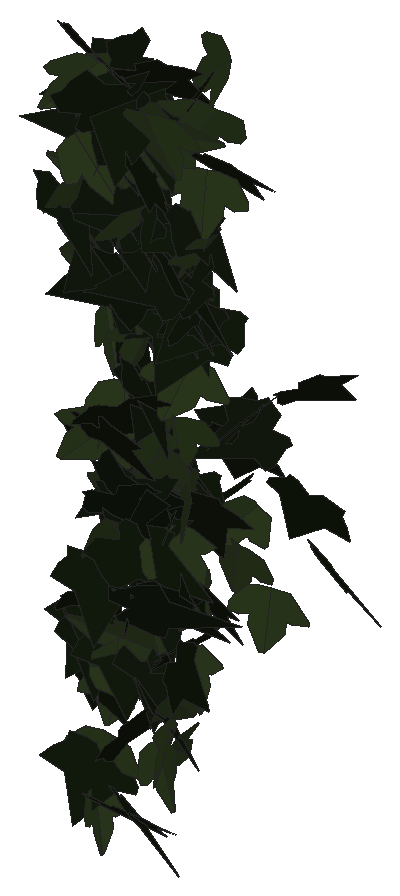
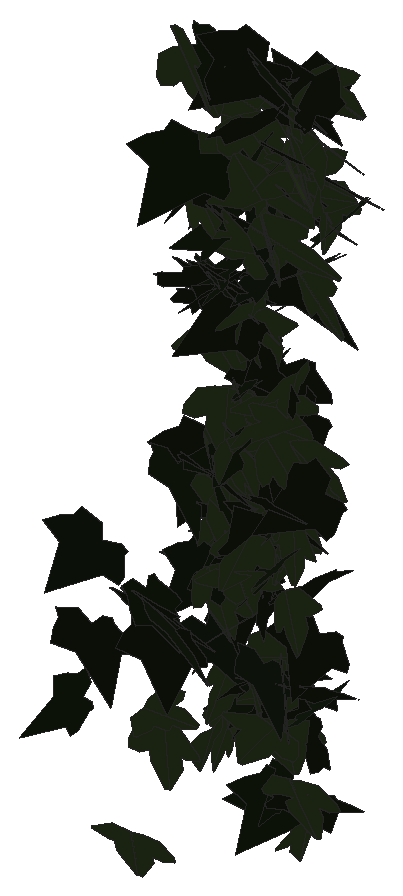
# SketchUp Ruby script. Lengths in inches.
U = 1.inch
M = Sketchup.active_model
def pt(a) = Geom::Point3d.new(a.map { |v| v * U })
def face(e, loops, mat)
  f = e.add_face(loops[0].map { |a| pt(a) })
  loops[1..].each { |l| e.add_face(l.map { |a| pt(a) }).erase! }
  f.material = f.back_material = mat if mat
  f
end
# faces: each face lists its corners as indices into pts; further lists are holes
def faces(e, pts, list, mat = nil) = list.each { |f| face(e, (f[0].is_a?(Array) ? f : [f]).map { |l| l.map { |i| pts[i] } }, mat) }
# xy, xz, yz: faces in a plane at the given z, y or x. An outline is a flat list of corners, or four numbers for a rectangle; further outlines are holes
def ring(l) = l.size == 4 ? [[l[0], l[1]], [l[2], l[1]], [l[2], l[3]], [l[0], l[3]]] : l.each_slice(2).to_a
def flat(e, list, mat, &to3) = list.each { |f| face(e, (f[0].is_a?(Array) ? f : [f]).map { |l| ring(l).map { |u, v| to3.(u, v) } }, mat) }
def xy(e, z, list, mat = nil) = flat(e, list, mat) { |x, y| [x, y, z] }
def xz(e, y, list, mat = nil) = flat(e, list, mat) { |x, z| [x, y, z] }
def yz(e, x, list, mat = nil) = flat(e, list, mat) { |y, z| [x, y, z] }
def lines(e, pts, list) = list.each { |a, b| e.add_line(pt(pts[a]), pt(pts[b])) }
# prism: a flat outline (further loops are holes) pulled along v
def prism(e, loops, v, mat = nil)
  f = face(e, loops, mat); d = Geom::Vector3d.new(v.map { |x| x * U })
  f.pushpull(f.normal.samedirection?(d) ? d.length : -d.length)
end
def box(e, o, s, mat = nil) = prism(e, [[o, [o[0] + s[0], o[1], o[2]], [o[0] + s[0], o[1] + s[1], o[2]], [o[0], o[1] + s[1], o[2]]]], [0, 0, s[2]], mat)
def at(x, y, z, deg = 0) = Geom::Transformation.translation(pt([x, y, z])) * Geom::Transformation.rotation(ORIGIN, Z_AXIS, deg.degrees)
def axes(o, x, y, z) = Geom::Transformation.new([*x, 0, *y, 0, *z, 0, *pt(o).to_a, 1])
def part(name) = M.definitions.add(name)
# library, detail: a bought-in or finely detailed component or shape, given as its bounding box
def library(name, o, s) = part(name).tap { |d| box(d.entities, o, s) }
def detail(e, o, s) = box(e.add_group.entities, o, s)
def put(e, d, t, mat = nil) = e.add_instance(d, t).tap { |i| i.material = mat if mat }
def group(e, t, mat = nil) = e.add_group.tap { |g| g.transformation = t; g.material = mat if mat }.entities
root = M.entities
M.materials.add("1026 AP 7946 SUNNY SIDE UP").color = [254, 231, 186]
M.materials.add("efeu1").color = [18, 25, 13]
M.materials.add("efeu2").color = [43, 57, 29]
c1 = part("ivyleaf_10")
p = [[0,0.5,-0.03],[-0.0625,2.02,-0.43],[-0.19,2.01,-0.46],[-0.54,1.05,-0.29],[-0.52,0.625,-0.18],[-0.83,0.76,-0.28],
  [-1.16,0.64,-0.33],[-1.15,0.33,-0.24],[-0.77,-0.39,0.02],[-0.3,-0.51,0.16],[0.04,-0.48,0.23],[-0.02,2.01,-0.4375],
  [-0.06,2.01,-0.43],[0.04,-0.49,0.23],[0.67,-0.49,0.14],[1.38,0.36,-0.2],[1.375,0.51,-0.24],[0.81,0.65,-0.19],
  [0.62,0.59,-0.15],[0.6,1.09,-0.28],[0.5,1.23,-0.31]]
faces(c1.entities,p,[[0,1,2,3,4,5,6,7,8,9,10],[11,12,0,13,14,15,16,17,18,19,20]],"efeu2")
c2 = part("ivyleaf_9")
p = [[1.54,2.16,1.25],[1.36,2.04,1.19],[-0.21,0.99,0.68],[-0.71,1.11,0.82],[-0.85,0.86,0.67],[-0.8,0.17,0.21],
  [-0.9,-0.01,0.1],[-0.67,-0.16,-0.02],[-0.08,-0.08,-0.05],[-0.03,-0.6,-0.4],[0.65,-0.88,-0.66],[0.83,-0.6,-0.49],
  [1.29,-0.42,-0.43],[1.8125,-0.07,-0.26],[1.21,0.44,0.15]]
faces(c2.entities,p,[[0,1,2,3,4,5,6,7,8,9,10,11,12,13,14]],"efeu1")
put(root,c1,axes([136.3125,212.4,287.8],[0.22711,-0.11423,-0.31893],[-0.31523,0.23716,-0.18551],[0.41092,0.24506,0.03395]),"1026 AP 7946 SUNNY SIDE UP")
put(root,c2,axes([136.11,212.92,282.05],[-0.39568,-0.19677,-0.00291],[0.06839,-0.05292,-0.32174],[0.30176,-0.24602,0.0691]),"1026 AP 7946 SUNNY SIDE UP")
put(root,c2,axes([135.93,212.8,281.74],[-0.01762,-0.28672,0.14922],[0.03799,-0.1469,-0.29519],[0.50484,0.00105,0.02742]),"1026 AP 7946 SUNNY SIDE UP")
put(root,c2,axes([136.11,212.5,282.66],[0.19885,0.2925,0.05494],[0.06419,0.03851,-0.32729],[-0.46262,0.13107,-0.0218]),"1026 AP 7946 SUNNY SIDE UP")
put(root,c2,axes([136.56,212.64,289.74],[-0.41749,0.17956,0.16578],[-0.29275,-0.0028,-0.31525],[-0.23923,-0.30993,0.09647]),"1026 AP 7946 SUNNY SIDE UP")
put(root,c2,axes([136.4375,215.3,284.04],[-0.17558,0.27212,0.14792],[-0.13121,0.11854,-0.30085],[-0.46449,-0.13635,0.02907]),"1026 AP 7946 SUNNY SIDE UP")
put(root,c1,axes([136.02,212.76,290.125],[-0.38951,0.18272,-0.18147],[0.16298,-0.1534,-0.31315],[-0.36553,-0.26311,0.05375]),"1026 AP 7946 SUNNY SIDE UP")
put(root,c2,axes([136.35,212.9375,282.23],[0.0418,-0.02393,-0.32843],[-0.44677,0.14457,-0.03476],[0.22996,0.28523,-0.00783]),"1026 AP 7946 SUNNY SIDE UP")
put(root,c2,axes([135.87,212.71,284.94],[0.55171,-0.05991,0.00291],[-0.0043,-0.03472,-0.36515],[0.09424,0.34916,-0.03369]),"1026 AP 7946 SUNNY SIDE UP")
put(root,c2,axes([135.95,212.21,288.77],[0.13325,-0.34559,0.0192],[-0.00393,-0.02182,-0.36662],[0.54436,0.08444,-0.00734]),"1026 AP 7946 SUNNY SIDE UP")
put(root,c1,axes([136.2,212.11,289.04],[-0.0567,-0.33283,-0.13417],[0.05703,0.12491,-0.34347],[0.558,-0.04658,0.02147]),"1026 AP 7946 SUNNY SIDE UP")
put(root,c2,axes([136.57,212.78,290.51],[-0.50445,0.15238,0.04087],[-0.09305,-0.0353,-0.36136],[-0.22907,-0.32122,0.05677]),"1026 AP 7946 SUNNY SIDE UP")
put(root,c1,axes([136.38,212.21,290.72],[0.30855,0.18135,-0.23522],[-0.30332,-0.12727,-0.27444],[-0.3455,0.27369,0.03088]),"1026 AP 7946 SUNNY SIDE UP")
put(root,c1,axes([136.21,212.88,286.625],[0.04732,0.33528,-0.05256],[-0.00894,-0.05263,-0.3471],[-0.53365,0.03061,0.00116]),"1026 AP 7946 SUNNY SIDE UP")
put(root,c2,axes([135.9375,212.75,281.33],[0.06984,-0.05533,-0.32343],[0.49967,-0.01336,0.04871],[-0.0333,-0.31648,0.05258]),"1026 AP 7946 SUNNY SIDE UP")
put(root,c2,axes([136.31,212.5625,280.15],[-0.35995,-0.22147,-0.03792],[0.05886,0.01237,-0.32759],[0.34775,-0.23133,0.01619]),"1026 AP 7946 SUNNY SIDE UP")
put(root,c1,axes([136.45,212.43,285.25],[0.45702,0.00054,-0.18527],[-0.28272,0.0078,-0.2993],[0.00573,0.3417,0.00912]),"1026 AP 7946 SUNNY SIDE UP")
put(root,c2,axes([136.38,215.33,283.78],[0.36414,0.10931,-0.20524],[-0.29646,-0.06793,-0.26376],[-0.20098,0.29825,0.01721]),"1026 AP 7946 SUNNY SIDE UP")
put(root,c1,axes([136.43,212.68,284.16],[-0.45237,0.14785,0.07414],[-0.13808,-0.01749,-0.32859],[-0.21792,-0.29584,0.05431]),"1026 AP 7946 SUNNY SIDE UP")
put(root,c1,axes([136.36,212.77,283.15],[-0.05788,-0.32062,-0.01386],[0.01286,0.01077,-0.33233],[0.5043,-0.03707,0.00688]),"1026 AP 7946 SUNNY SIDE UP")
put(root,c1,axes([136.34,212.64,280.33],[0.48967,-0.00134,-0.07543],[-0.11421,0.0349,-0.31874],[0.0146,0.318,0.03655]),"1026 AP 7946 SUNNY SIDE UP")
put(root,c2,axes([136,212.71,290.64],[0.02921,-0.17516,0.31941],[0.26543,-0.27013,-0.16868],[0.49458,0.15532,0.07166]),"1026 AP 7946 SUNNY SIDE UP")
put(root,c2,axes([136.53,213.08,282.3],[-0.0458,0.31236,0.06995],[-0.01903,0.06527,-0.32275],[-0.50169,-0.03099,0.00586]),"1026 AP 7946 SUNNY SIDE UP")
put(root,c1,axes([136.37,212.65,289.99],[0.29784,-0.30633,-0.0179],[0.01599,0.02464,-0.37023],[0.48204,0.18846,0.02334]),"1026 AP 7946 SUNNY SIDE UP")
put(root,c1,axes([136.82,212.36,289.03],[-0.10399,-0.03302,-0.37806],[-0.57717,0.03614,0.06504],[0.04697,0.37095,-0.03778]),"1026 AP 7946 SUNNY SIDE UP")
put(root,c1,axes([136.3125,212.61,290.47],[0.00072,-0.11466,0.35277],[0.1722,-0.32694,-0.11462],[0.5421,0.10401,0.03594]),"1026 AP 7946 SUNNY SIDE UP")
put(root,c1,axes([136.78,212.65,288.48],[0.20804,-0.05926,-0.35938],[-0.53558,0.07823,-0.14646],[0.14878,0.36448,-0.0247]),"1026 AP 7946 SUNNY SIDE UP")
put(root,c1,axes([136.55,215.2,282.19],[-0.4989,0.05063,0.08616],[-0.13581,-0.01421,-0.32994],[-0.07119,-0.32774,0.02565]),"1026 AP 7946 SUNNY SIDE UP")
put(root,c1,axes([136.4,212.8,281.29],[0.39938,0.19612,-0.03382],[-0.08539,0.01534,-0.32721],[-0.30108,0.25579,0.04794]),"1026 AP 7946 SUNNY SIDE UP")
put(root,c1,axes([136.54,215.4,282.68],[0.18051,0.15225,-0.26543],[-0.24645,-0.20559,-0.19764],[-0.40226,0.19428,0.00198]),"1026 AP 7946 SUNNY SIDE UP")
put(root,c1,axes([136.2,213.4,281.5625],[0.41864,0.08276,0.15999],[0.2167,0.07574,-0.28538],[-0.17103,0.29853,0.03004]),"1026 AP 7946 SUNNY SIDE UP")
put(root,c1,axes([136.47,212.58,289.62],[0.23919,-0.31924,0.07365],[0.02174,-0.07449,-0.36421],[0.51458,0.15154,-0.01885]),"1026 AP 7946 SUNNY SIDE UP")
put(root,c1,axes([136.375,216,281.06],[0.50983,0.03135,0.03273],[0.0544,-0.03145,-0.33388],[-0.04402,0.32425,-0.03362]),"1026 AP 7946 SUNNY SIDE UP")
put(root,c1,axes([136.4375,212.36,279.63],[0.04171,0.31122,-0.0649],[-0.0065,-0.06465,-0.32215],[-0.4998,0.02681,-0.00123]),"1026 AP 7946 SUNNY SIDE UP")
put(root,c2,axes([136.53,212.49,287.9],[-0.28062,-0.21055,0.21638],[-0.05922,-0.22828,-0.26853],[0.46521,-0.15606,0.09634]),"1026 AP 7946 SUNNY SIDE UP")
put(root,c1,axes([136.89,212.55,282.11],[-0.15009,0.0224,-0.32404],[-0.49191,-0.04909,0.09387],[-0.06393,0.32515,0.03845]),"1026 AP 7946 SUNNY SIDE UP")
put(root,c2,axes([136.72,215.27,284.32],[-0.1906,0.28286,-0.11514],[0.04144,-0.11182,-0.3171],[-0.47737,-0.12265,0.01844]),"1026 AP 7946 SUNNY SIDE UP")
put(root,c2,axes([136.89,212.25,287.76],[0.08438,-0.00333,-0.37536],[-0.51526,-0.16145,-0.04914],[-0.25048,0.331,-0.02535]),"1026 AP 7946 SUNNY SIDE UP")
put(root,c1,axes([136.38,212.15,289.58],[0.23375,0.32418,0.14353],[0.11799,0.11664,-0.36624],[-0.54097,0.16552,-0.01786]),"1026 AP 7946 SUNNY SIDE UP")
put(root,c1,axes([136.66,212.6875,285.29],[-0.14496,-0.30093,0.13342],[-0.02274,-0.13244,-0.32414],[0.5157,-0.09043,0.02321]),"1026 AP 7946 SUNNY SIDE UP")
put(root,c2,axes([136.51,212.27,283.17],[-0.11539,-0.32614,0.0352],[-0.00514,-0.03618,-0.34457],[0.51592,-0.07331,0.00444]),"1026 AP 7946 SUNNY SIDE UP")
put(root,c2,axes([136.4,212.85,283.83],[0.17585,-0.31037,0.00954],[0.00809,-0.00986,-0.33992],[0.48827,0.11194,0.0022]),"1026 AP 7946 SUNNY SIDE UP")
put(root,c2,axes([136.88,212.81,284.51],[-0.51971,-0.00684,0.00555],[-0.00759,-0.02808,-0.33952],[0.01144,-0.32937,0.02689]),"1026 AP 7946 SUNNY SIDE UP")
put(root,c2,axes([136.96,215.29,284.15],[-0.51099,0.04314,0.051],[-0.08307,-0.02544,-0.33628],[-0.06082,-0.3277,0.03086]),"1026 AP 7946 SUNNY SIDE UP")
put(root,c2,axes([136.88,212.65,290.91],[-0.49048,0.15024,-0.11639],[0.12366,-0.09628,-0.35351],[-0.26936,-0.31778,0.04964]),"1026 AP 7946 SUNNY SIDE UP")
put(root,c1,axes([136.69,212.27,284.03],[-0.07167,-0.3198,-0.2423],[0.08889,0.22726,-0.33086],[0.61614,-0.06999,0.01955]),"1026 AP 7946 SUNNY SIDE UP")
put(root,c2,axes([136.51,212.46,290.5],[-0.31983,-0.12909,-0.27626],[0.43459,0.03623,-0.23437],[0.17075,-0.33403,0.07907]),"1026 AP 7946 SUNNY SIDE UP")
put(root,c1,axes([136.54,212.41,281.68],[-0.00004,0.04067,0.34352],[0.1383,0.32158,-0.03854],[-0.5094,0.0873,-0.01049]),"1026 AP 7946 SUNNY SIDE UP")
put(root,c1,axes([136.77,212.73,288.61],[0.20674,-0.32517,-0.03944],[0.00088,0.0395,-0.36076],[0.5145,0.13059,0.01646]),"1026 AP 7946 SUNNY SIDE UP")
put(root,c2,axes([136.64,212.64,281.97],[-0.20693,-0.28592,-0.07174],[0.106,0.04317,-0.32108],[0.44981,-0.14171,0.04266]),"1026 AP 7946 SUNNY SIDE UP")
put(root,c2,axes([136.51,212.59,289.77],[0.25727,-0.37368,-0.10031],[-0.08449,0.08037,-0.41943],[0.60045,0.17141,-0.01604]),"1026 AP 7946 SUNNY SIDE UP")
put(root,c2,axes([136.53,212.83,286.61],[-0.13587,-0.03758,-0.33807],[0.51895,-0.00347,-0.08919],[0.00975,-0.33912,0.03637]),"1026 AP 7946 SUNNY SIDE UP")
put(root,c2,axes([136.53,211.95,290.28],[0.03045,0.02938,0.3747],[0.54116,0.11908,-0.0281],[-0.18991,0.34404,-0.02]),"1026 AP 7946 SUNNY SIDE UP")
put(root,c2,axes([136.63,212.52,284.25],[0.21093,-0.30298,0.00086],[-0.01608,-0.00732,-0.34116],[0.47614,0.13397,-0.0119]),"1026 AP 7946 SUNNY SIDE UP")
put(root,c1,axes([136.79,212.46,285.87],[0.39465,0.22971,-0.04215],[-0.02282,-0.04651,-0.34988],[-0.36653,0.25023,-0.02359]),"1026 AP 7946 SUNNY SIDE UP")
put(root,c1,axes([136.66,212.41,285.53],[0.16685,0.1384,0.30179],[0.23709,0.25082,-0.17735],[-0.44966,0.1836,0.01847]),"1026 AP 7946 SUNNY SIDE UP")
put(root,c2,axes([136.66,212.01,285.57],[0.52368,-0.04702,0.00067],[-0.00496,-0.0289,-0.34538],[0.07379,0.33179,-0.02799]),"1026 AP 7946 SUNNY SIDE UP")
put(root,c2,axes([137.39,212.24,288.92],[-0.48703,0.16453,0.16946],[-0.26493,0.02802,-0.35758],[-0.25076,-0.34915,0.04865]),"1026 AP 7946 SUNNY SIDE UP")
put(root,c2,axes([136.97,212.84,283.96],[-0.20102,-0.11789,0.29019],[0.28106,0.21959,0.17911],[-0.39049,0.21874,-0.02047]),"1026 AP 7946 SUNNY SIDE UP")
put(root,c2,axes([136.83,212.76,283.11],[-0.08175,-0.00145,-0.33677],[0.40047,-0.20768,-0.042],[-0.32222,-0.25774,0.03325]),"1026 AP 7946 SUNNY SIDE UP")
put(root,c1,axes([136.98,212.79,281.79],[0.22839,-0.28895,-0.03209],[0.00184,0.03358,-0.33256],[0.4567,0.14436,0.01739]),"1026 AP 7946 SUNNY SIDE UP")
put(root,c1,axes([136.95,212.94,283.92],[-0.27695,-0.23603,-0.14639],[0.1613,0.09864,-0.30205],[0.40089,-0.20275,0.0204]),"1026 AP 7946 SUNNY SIDE UP")
put(root,c2,axes([136.9,212.11,279.82],[0.5028,0.10917,-0.06421],[-0.14578,0.08753,-0.3283],[-0.1342,0.31393,0.11606]),"1026 AP 7946 SUNNY SIDE UP")
put(root,c2,axes([136.95,212.36,290.54],[-0.4233,-0.28342,-0.12915],[0.17244,0.06593,-0.40092],[0.45469,-0.28886,0.03181]),"1026 AP 7946 SUNNY SIDE UP")
put(root,c1,axes([137.07,212.58,286.95],[-0.1322,-0.33121,0.09048],[0.00977,-0.09382,-0.35138],[0.53947,-0.07946,0.02854]),"1026 AP 7946 SUNNY SIDE UP")
put(root,c2,axes([136.93,212.83,283.18],[-0.09125,-0.17865,0.27422],[-0.03727,-0.2684,-0.19174],[0.50402,-0.05219,0.03547]),"1026 AP 7946 SUNNY SIDE UP")
put(root,c1,axes([136.93,212.7,289.09],[0.36994,0.25285,-0.18288],[0.1631,0.14744,0.35596],[0.45896,-0.2562,0.02091]),"1026 AP 7946 SUNNY SIDE UP")
put(root,c2,axes([136.8125,212.625,287.27],[0.20173,-0.29649,-0.1223],[0.01356,0.12934,-0.32706],[0.50102,0.11588,0.05809]),"1026 AP 7946 SUNNY SIDE UP")
put(root,c2,axes([137.13,211.9,286.04],[0.22753,0.33761,-0.05904],[-0.01881,-0.05928,-0.37854],[-0.53863,0.14468,-0.01172]),"1026 AP 7946 SUNNY SIDE UP")
put(root,c1,axes([137.02,212.98,283.41],[0.43556,0.15949,-0.05077],[-0.04212,-0.05354,-0.32788],[-0.25951,0.27638,-0.03201]),"1026 AP 7946 SUNNY SIDE UP")
put(root,c1,axes([137,213.66,281.38],[0.03448,0.31829,-0.03738],[0.00178,-0.03826,-0.32888],[-0.50405,0.02164,-0.00372]),"1026 AP 7946 SUNNY SIDE UP")
put(root,c2,axes([137.12,211.97,281.04],[-0.10688,0.15174,-0.30658],[-0.1888,0.27324,0.17289],[0.49144,0.13797,-0.00026]),"1026 AP 7946 SUNNY SIDE UP")
put(root,c2,axes([136.89,212.29,289.02],[-0.35433,-0.15468,-0.3046],[0.43712,0.10842,-0.27689],[0.288,-0.35486,0.04551]),"1026 AP 7946 SUNNY SIDE UP")
put(root,c1,axes([137.28,212.5,289.84],[-0.39572,-0.18881,0.18091],[-0.10722,-0.18936,-0.30964],[0.3922,-0.24227,0.09789]),"1026 AP 7946 SUNNY SIDE UP")
put(root,c2,axes([136.9,212.53,287.89],[0.40729,-0.20309,-0.11978],[-0.12458,0.08526,-0.33812],[0.34528,0.27033,0.01929]),"1026 AP 7946 SUNNY SIDE UP")
put(root,c2,axes([137.02,212.79,281.8],[-0.05973,-0.31869,0.04948],[-0.01134,-0.04933,-0.33093],[0.50708,-0.03865,-0.00157]),"1026 AP 7946 SUNNY SIDE UP")
put(root,c2,axes([136.82,212.3,284.42],[0.02033,-0.01933,0.38957],[0.27881,-0.33414,-0.02579],[0.52627,0.17777,-0.00139]),"1026 AP 7946 SUNNY SIDE UP")
put(root,c1,axes([137.25,212.82,285.13],[-0.14349,-0.30588,0.10572],[-0.00999,-0.10672,-0.3286],[0.50809,-0.08849,0.0234]),"1026 AP 7946 SUNNY SIDE UP")
put(root,c2,axes([137.02,212.74,290.18],[-0.04167,-0.34441,-0.09744],[0.00837,0.0925,-0.35532],[0.56074,-0.02697,-0.00194]),"1026 AP 7946 SUNNY SIDE UP")
put(root,c2,axes([137.02,212.97,282.75],[-0.00415,-0.31644,0.06298],[0.02756,-0.06298,-0.32586],[0.50656,0.00083,0.01825]),"1026 AP 7946 SUNNY SIDE UP")
put(root,c2,axes([137.01,212.37,288.48],[0.44998,-0.19191,-0.11613],[-0.16701,0.0416,-0.3539],[0.30656,0.30435,-0.02233]),"1026 AP 7946 SUNNY SIDE UP")
put(root,c1,axes([137.13,212.62,287.26],[0.07401,0.34029,-0.03045],[-0.00288,-0.03154,-0.35408],[-0.53735,0.04704,-0.0023]),"1026 AP 7946 SUNNY SIDE UP")
put(root,c1,axes([137.27,212.13,288.88],[-0.14542,-0.37151,-0.0488],[0.0298,0.04191,-0.39408],[0.58773,-0.09405,0.00791]),"1026 AP 7946 SUNNY SIDE UP")
put(root,c2,axes([137.1,211.96,284.67],[0.47798,0.23223,0.01961],[0.05161,-0.01388,-0.39288],[-0.36257,0.30418,-0.03007]),"1026 AP 7946 SUNNY SIDE UP")
put(root,c1,axes([137.3125,212.79,283.79],[0.22488,-0.29154,-0.0274],[-0.04996,0.01212,-0.33361],[0.45737,0.14467,-0.02297]),"1026 AP 7946 SUNNY SIDE UP")
put(root,c2,axes([137.09,212.43,290.87],[0.46649,0.17233,0.09531],[0.12449,0.04595,-0.35318],[-0.28045,0.30705,0.00176]),"1026 AP 7946 SUNNY SIDE UP")
put(root,c2,axes([137,212.24,279.85],[0.30853,-0.24011,0.08468],[0.0687,-0.07214,-0.31966],[0.39382,0.2007,-0.01058]),"1026 AP 7946 SUNNY SIDE UP")
put(root,c2,axes([137.46,212.84,284.25],[-0.44924,-0.15779,0.02911],[-0.02144,-0.03545,-0.3355],[0.25139,-0.28499,0.02341]),"1026 AP 7946 SUNNY SIDE UP")
put(root,c2,axes([137.2,212.49,286.03],[-0.07552,-0.25079,0.23948],[-0.01847,-0.23483,-0.26326],[0.5389,-0.04319,0.02453]),"1026 AP 7946 SUNNY SIDE UP")
put(root,c1,axes([137.45,212.79,284.5],[-0.50717,-0.0119,0.05678],[-0.08307,-0.04921,-0.32932],[0.0313,-0.32351,0.04606]),"1026 AP 7946 SUNNY SIDE UP")
put(root,c1,axes([137.38,212.94,284.31],[-0.0085,-0.26128,0.20233],[0.03334,-0.19777,-0.26958],[0.51429,0.0085,0.02082]),"1026 AP 7946 SUNNY SIDE UP")
put(root,c2,axes([137.2,212.7,287.14],[0.27835,0.22059,0.20921],[0.23652,0.13699,-0.28937],[-0.4063,0.23087,-0.02513]),"1026 AP 7946 SUNNY SIDE UP")
put(root,c2,axes([137.16,212.39,286.2],[0.14282,-0.30675,0.12433],[0.02655,-0.1225,-0.32981],[0.51866,0.09074,-0.01736]),"1026 AP 7946 SUNNY SIDE UP")
put(root,c2,axes([137.23,212.19,289.68],[0.39148,-0.23588,-0.19102],[-0.21519,0.12318,-0.35257],[0.41837,0.28407,-0.00261]),"1026 AP 7946 SUNNY SIDE UP")
put(root,c2,axes([137.64,212.34,285.13],[-0.45275,0.15205,-0.08228],[0.08058,-0.07449,-0.33325],[-0.25843,-0.28961,0.04024]),"1026 AP 7946 SUNNY SIDE UP")
put(root,c1,axes([137.73,212.16,285.45],[-0.43104,0.08161,0.23791],[-0.36917,0.00875,-0.29083],[-0.10727,-0.35803,0.04491]),"1026 AP 7946 SUNNY SIDE UP")
put(root,c2,axes([137.17,212.57,281.42],[0.29687,-0.2595,0.04365],[0.01445,-0.04743,-0.33021],[0.41356,0.18793,-0.01979]),"1026 AP 7946 SUNNY SIDE UP")
put(root,c2,axes([137.09,212.07,283.91],[0.08034,-0.1208,-0.33634],[0.27563,0.29329,-0.08199],[0.47175,-0.15079,0.10519]),"1026 AP 7946 SUNNY SIDE UP")
put(root,c2,axes([137.55,212.4,282.98],[0.13991,0.30905,-0.05065],[-0.01625,-0.05001,-0.33159],[-0.49224,0.08949,-0.00345]),"1026 AP 7946 SUNNY SIDE UP")
put(root,c1,axes([137.55,212.875,283.16],[-0.17215,-0.30262,0.05471],[0.00645,-0.05962,-0.33097],[0.48354,-0.10694,0.02389]),"1026 AP 7946 SUNNY SIDE UP")
put(root,c1,axes([137.12,212.6875,288.13],[0.24644,-0.01692,0.32335],[0.48021,-0.07525,-0.16167],[0.1176,0.34275,-0.01742]),"1026 AP 7946 SUNNY SIDE UP")
put(root,c2,axes([137.71,212.78,282.33],[-0.15751,0.27801,-0.14261],[0.01319,-0.14461,-0.30286],[-0.48927,-0.0934,0.03775]),"1026 AP 7946 SUNNY SIDE UP")
put(root,c2,axes([137.42,215.42,284.89],[0.30617,0.23613,0.13398],[0.12203,0.10281,-0.31466],[-0.40489,0.20955,0.00648]),"1026 AP 7946 SUNNY SIDE UP")
put(root,c1,axes([137.55,212.81,282.97],[0.47717,-0.09526,-0.06626],[-0.07017,0.06808,-0.3231],[0.16603,0.30253,0.05388]),"1026 AP 7946 SUNNY SIDE UP")
put(root,c2,axes([137.45,212.91,284.66],[-0.19979,-0.01155,-0.31462],[0.40235,-0.18474,-0.10358],[-0.26257,-0.2743,0.08067]),"1026 AP 7946 SUNNY SIDE UP")
put(root,c2,axes([137.93,212.16,288.125],[-0.50061,0.09958,0.11546],[-0.18525,-0.00562,-0.3414],[-0.14472,-0.33729,0.03763]),"1026 AP 7946 SUNNY SIDE UP")
put(root,c2,axes([137.22,212.82,285.14],[0.36778,-0.23684,0.04913],[0.06516,-0.02797,-0.34294],[0.37469,0.23734,0.01141]),"1026 AP 7946 SUNNY SIDE UP")
put(root,c1,axes([137.61,212.54,285.65],[-0.48547,-0.1519,-0.00551],[0.02566,-0.02305,-0.35344],[0.23757,-0.30791,0.02692]),"1026 AP 7946 SUNNY SIDE UP")
put(root,c1,axes([137.66,212.47,280.77],[0.05587,0.16418,0.28596],[-0.20879,0.261,-0.14047],[-0.46073,-0.09837,0.09833]),"1026 AP 7946 SUNNY SIDE UP")
put(root,c1,axes([137.65,212.26,285.76],[0.19182,-0.31404,-0.10558],[-0.06972,0.09077,-0.34644],[0.51385,0.12955,-0.00759]),"1026 AP 7946 SUNNY SIDE UP")
put(root,c2,axes([137.7,215.22,283.43],[0.32913,0.05981,-0.26222],[-0.36739,-0.10451,-0.22356],[-0.18568,0.31281,-0.02246]),"1026 AP 7946 SUNNY SIDE UP")
put(root,c1,axes([137.52,212.17,290.32],[-0.54646,0.02181,-0.08653],[0.12844,-0.03632,-0.35759],[-0.04662,-0.35572,0.0291]),"1026 AP 7946 SUNNY SIDE UP")
put(root,c2,axes([137.89,212.49,287.53],[-0.40194,0.23741,0.00528],[-0.02841,-0.01392,-0.35873],[-0.37227,-0.25527,0.02168]),"1026 AP 7946 SUNNY SIDE UP")
put(root,c1,axes([137.6,212.49,281.57],[-0.09779,-0.25046,-0.23976],[0.09096,0.22396,-0.26455],[0.52831,-0.08492,0.00117]),"1026 AP 7946 SUNNY SIDE UP")
put(root,c2,axes([137.39,212.78,287.74],[0.22782,-0.30472,0.06968],[0.02079,-0.07041,-0.34752],[0.49097,0.14438,-0.01761]),"1026 AP 7946 SUNNY SIDE UP")
put(root,c2,axes([137.67,212.89,284.74],[-0.44029,-0.057,-0.16658],[0.26618,-0.04669,-0.28588],[0.03961,-0.31979,0.06946]),"1026 AP 7946 SUNNY SIDE UP")
put(root,c2,axes([137.37,212.22,283.15],[0.4954,0.07178,0.10577],[0.16691,-0.00749,-0.33155],[-0.10361,0.33116,-0.0284]),"1026 AP 7946 SUNNY SIDE UP")
put(root,c2,axes([137.97,212.67,287.5625],[-0.54036,0.03951,0.02397],[-0.04294,-0.0371,-0.3542],[-0.05769,-0.34242,0.03909]),"1026 AP 7946 SUNNY SIDE UP")
put(root,c2,axes([137.25,212.07,282.96],[0.29317,0.00977,0.3106],[0.47419,-0.00157,-0.19212],[-0.00598,0.35444,-0.00734]),"1026 AP 7946 SUNNY SIDE UP")
put(root,c1,axes([137.61,212.39,281.04],[0.08849,-0.23106,0.24649],[0.1729,-0.21749,-0.24297],[0.49519,0.11723,0.04079]),"1026 AP 7946 SUNNY SIDE UP")
put(root,c2,axes([137.53,212.83,287.51],[0.05718,-0.34122,-0.03386],[-0.01695,0.02995,-0.35325],[0.53847,0.03717,-0.00752]),"1026 AP 7946 SUNNY SIDE UP")
put(root,c1,axes([137.78,212.53,286.53],[0.45366,0.15817,-0.10903],[-0.1336,-0.06676,-0.33891],[-0.26866,0.30029,-0.01558]),"1026 AP 7946 SUNNY SIDE UP")
put(root,c2,axes([137.83,212.61,287.22],[-0.39911,-0.2349,-0.01691],[0.04379,-0.00794,-0.35542],[0.36752,-0.25415,0.02398]),"1026 AP 7946 SUNNY SIDE UP")
put(root,c1,axes([137.625,212.36,283.93],[0.27713,0.29533,0.15304],[0.11386,0.12783,-0.35354],[-0.50598,0.19052,0.00426]),"1026 AP 7946 SUNNY SIDE UP")
put(root,c1,axes([137.99,212.97,291.08],[0.25279,-0.28407,-0.23083],[-0.20619,0.18088,-0.33453],[0.52853,0.20643,-0.0201]),"1026 AP 7946 SUNNY SIDE UP")
put(root,c1,axes([137.51,212.23,280.78],[0.2955,-0.08027,0.29697],[0.39163,-0.14768,-0.21017],[0.26204,0.31124,-0.02078]),"1026 AP 7946 SUNNY SIDE UP")
put(root,c2,axes([137.7,213.04,289.52],[0.57933,0.10314,-0.0883],[-0.16641,0.06711,-0.38248],[-0.13046,0.3724,0.0958]),"1026 AP 7946 SUNNY SIDE UP")
put(root,c2,axes([137.68,212.4375,288.88],[0.0228,-0.31386,-0.18131],[-0.02037,0.17379,-0.32263],[0.56408,0.01896,-0.00432]),"1026 AP 7946 SUNNY SIDE UP")
put(root,c2,axes([137.79,212.72,283.29],[-0.0617,-0.09257,0.32629],[-0.05542,-0.31649,-0.10147],[0.51669,-0.045,0.02808]),"1026 AP 7946 SUNNY SIDE UP")
put(root,c2,axes([138.24,212.21,288.22],[-0.4714,0.1627,0.05567],[-0.0912,0.00421,-0.35053],[-0.2532,-0.30444,0.02261]),"1026 AP 7946 SUNNY SIDE UP")
put(root,c1,axes([137.51,212.32,290.13],[-0.20482,-0.05321,0.33994],[0.51252,0.05961,0.14267],[-0.11843,0.34999,0.02953]),"1026 AP 7946 SUNNY SIDE UP")
put(root,c2,axes([137.99,212.61,290.86],[-0.30504,0.14761,-0.27012],[0.26242,-0.20798,-0.24825],[-0.39506,-0.25212,0.04366]),"1026 AP 7946 SUNNY SIDE UP")
put(root,c2,axes([137.77,212.72,283.22],[0.49036,-0.04779,-0.09363],[-0.14264,0.00609,-0.32489],[0.07485,0.32469,-0.00575]),"1026 AP 7946 SUNNY SIDE UP")
put(root,c2,axes([138.1,212.76,287.49],[-0.41897,-0.2085,0.07944],[-0.07577,-0.06522,-0.34825],[0.3419,-0.26995,0.02017]),"1026 AP 7946 SUNNY SIDE UP")
put(root,c2,axes([137.97,212.12,282.36],[0.15672,-0.1536,-0.30531],[-0.30538,0.22375,-0.186],[0.42538,0.21722,-0.02105]),"1026 AP 7946 SUNNY SIDE UP")
put(root,c2,axes([137.74,215.43,282.4375],[0.4412,-0.17016,-0.06332],[-0.0749,0.03809,-0.33774],[0.27392,0.2845,0.00964]),"1026 AP 7946 SUNNY SIDE UP")
put(root,c2,axes([138.17,212.83,284.61],[-0.05835,0.3194,0.06965],[-0.0292,0.06404,-0.3307],[-0.51194,-0.04005,0.01092]),"1026 AP 7946 SUNNY SIDE UP")
put(root,c1,axes([138.02,212.66,289.42],[-0.50954,-0.14836,0.02757],[0.07427,-0.16182,-0.32569],[0.22536,-0.28211,0.16967]),"1026 AP 7946 SUNNY SIDE UP")
put(root,c1,axes([138.21,212.52,290.54],[-0.45441,-0.15373,0.13937],[-0.1684,-0.08775,-0.33674],[0.27553,-0.30717,0.02405]),"1026 AP 7946 SUNNY SIDE UP")
put(root,c2,axes([137.92,212.35,284.72],[0.52811,0.1296,-0.10442],[-0.12945,-0.069,-0.36967],[-0.22482,0.34418,-0.03241]),"1026 AP 7946 SUNNY SIDE UP")
put(root,c2,axes([137.73,212.35,288.18],[0.34976,-0.30814,0.00324],[-0.00058,-0.0063,-0.39152],[0.48458,0.2224,-0.0028]),"1026 AP 7946 SUNNY SIDE UP")
put(root,c1,axes([137.93,212.46,284.92],[0.17699,-0.27433,0.2178],[0.19307,-0.17799,-0.30409],[0.51083,0.16233,0.03947]),"1026 AP 7946 SUNNY SIDE UP")
put(root,c1,axes([138.11,212.45,288.5625],[-0.01655,-0.34619,0.07735],[0.00372,-0.07715,-0.35723],[0.55766,-0.00976,0.00468]),"1026 AP 7946 SUNNY SIDE UP")
put(root,c2,axes([137.91,212.48,288.97],[0.18367,-0.2767,-0.19189],[-0.1138,0.16992,-0.30842],[0.51057,0.13741,0.00028]),"1026 AP 7946 SUNNY SIDE UP")
